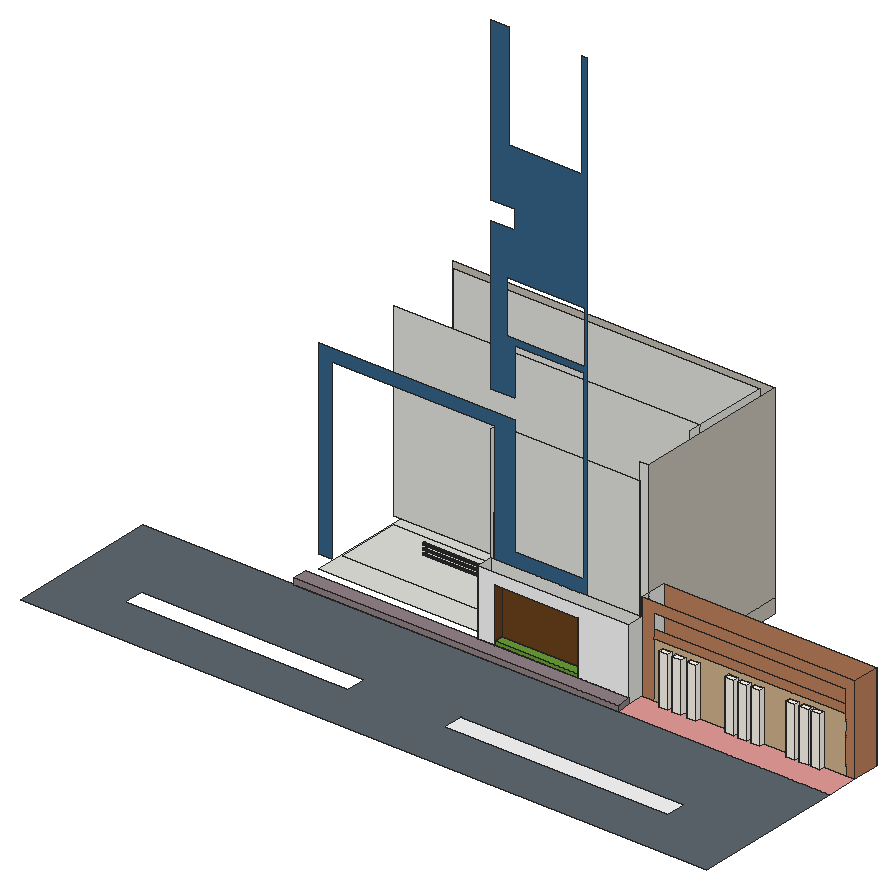
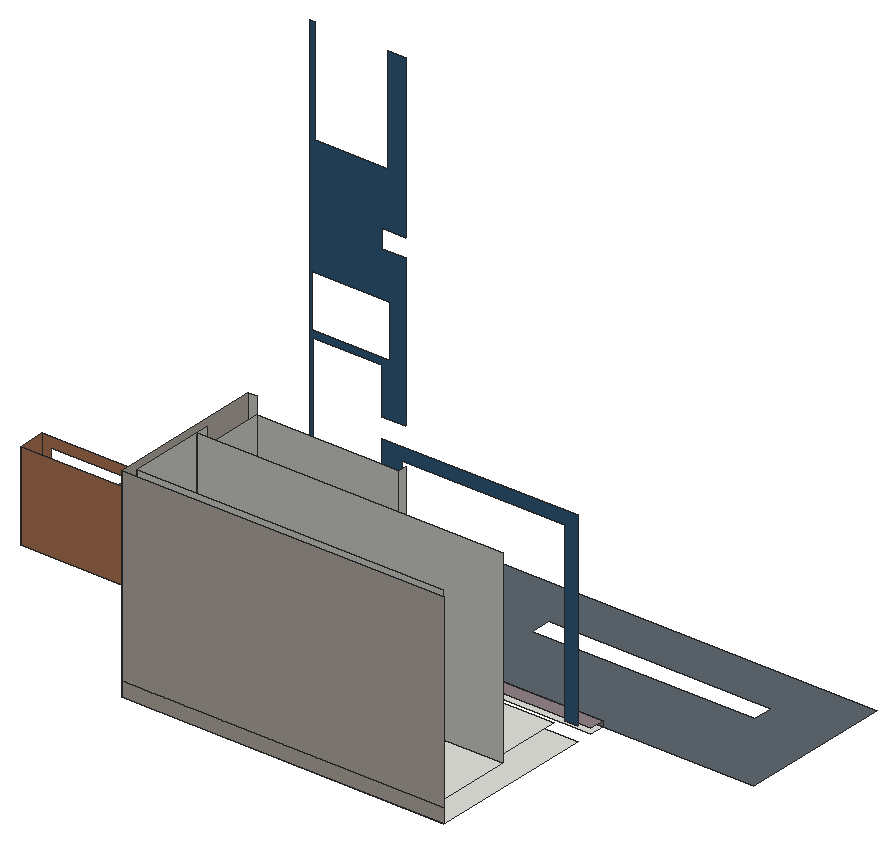
# SketchUp Ruby script. Lengths in inches.
U = 1.inch
M = Sketchup.active_model
def pt(a) = Geom::Point3d.new(a.map { |v| v * U })
def face(e, loops, mat)
  f = e.add_face(loops[0].map { |a| pt(a) })
  loops[1..].each { |l| e.add_face(l.map { |a| pt(a) }).erase! }
  f.material = f.back_material = mat if mat
  f
end
# faces: each face lists its corners as indices into pts; further lists are holes
def faces(e, pts, list, mat = nil) = list.each { |f| face(e, (f[0].is_a?(Array) ? f : [f]).map { |l| l.map { |i| pts[i] } }, mat) }
# xy, xz, yz: faces in a plane at the given z, y or x. An outline is a flat list of corners, or four numbers for a rectangle; further outlines are holes
def ring(l) = l.size == 4 ? [[l[0], l[1]], [l[2], l[1]], [l[2], l[3]], [l[0], l[3]]] : l.each_slice(2).to_a
def flat(e, list, mat, &to3) = list.each { |f| face(e, (f[0].is_a?(Array) ? f : [f]).map { |l| ring(l).map { |u, v| to3.(u, v) } }, mat) }
def xy(e, z, list, mat = nil) = flat(e, list, mat) { |x, y| [x, y, z] }
def xz(e, y, list, mat = nil) = flat(e, list, mat) { |x, z| [x, y, z] }
def yz(e, x, list, mat = nil) = flat(e, list, mat) { |y, z| [x, y, z] }
def lines(e, pts, list) = list.each { |a, b| e.add_line(pt(pts[a]), pt(pts[b])) }
# prism: a flat outline (further loops are holes) pulled along v
def prism(e, loops, v, mat = nil)
  f = face(e, loops, mat); d = Geom::Vector3d.new(v.map { |x| x * U })
  f.pushpull(f.normal.samedirection?(d) ? d.length : -d.length)
end
def box(e, o, s, mat = nil) = prism(e, [[o, [o[0] + s[0], o[1], o[2]], [o[0] + s[0], o[1] + s[1], o[2]], [o[0], o[1] + s[1], o[2]]]], [0, 0, s[2]], mat)
def at(x, y, z, deg = 0) = Geom::Transformation.translation(pt([x, y, z])) * Geom::Transformation.rotation(ORIGIN, Z_AXIS, deg.degrees)
def axes(o, x, y, z) = Geom::Transformation.new([*x, 0, *y, 0, *z, 0, *pt(o).to_a, 1])
def part(name) = M.definitions.add(name)
# library, detail: a bought-in or finely detailed component or shape, given as its bounding box
def library(name, o, s) = part(name).tap { |d| box(d.entities, o, s) }
def detail(e, o, s) = box(e.add_group.entities, o, s)
def put(e, d, t, mat = nil) = e.add_instance(d, t).tap { |i| i.material = mat if mat }
def group(e, t, mat = nil) = e.add_group.tap { |g| g.transformation = t; g.material = mat if mat }.entities
root = M.entities
M.materials.add("[0035_Tan]").color = [210, 180, 140]
M.materials.add("[0052_FloralWhite]").color = [255, 250, 240]
M.materials.add("[0100_SteelBlue]").color = [53, 99, 137]
M.materials.add("[Asphalt New]").color = [145, 130, 134]
M.materials.add("[Brick Basket]").color = [230, 156, 152]
M.materials.add("[Field Rectangle Tile]").color = [196, 189, 179]
M.materials.add("[Formica Laminate Dark]").color = [70, 74, 84]
M.materials.add("[Formica Speckled Grey]").color = [94, 105, 111]
M.materials.add("[Grass Dark Green]").color = [106, 157, 55]
M.materials.add("[Polished Concrete New]").color = [200, 200, 203]
M.materials.add("[Quartz Light Grey]").color = [251, 251, 252]
M.materials.add("[Wood Floor Parquet]").color = [107, 65, 28]
M.materials.add("[Wood Veneer 02]").color = [190, 128, 91]
xy(root,0,[[96.16,97.66,96.16,107.04,301.48,107.04,302.4,97.66],[205.34,107.04,205.34,117.35,301.48,117.35,301.48,107.04,269.29,107.04,269.29,112.73,216.35,112.73,216.35,107.04],[216.35,107.04,269.29,112.73],[315.22,114.1,320.97,117.35],[323.53,114.1,329.29,117.35],
  [332.72,114.1,338.47,117.35],[356.72,114.1,362.47,117.35],[365.41,114.1,371.16,117.35],[373.47,114.1,379.22,117.35],[396.03,114.1,401.79,117.35],
  [404.41,114.1,410.16,117.35],[411.78,114.1,417.54,117.35],[96.16,117.35,301.48,223.51],[301.48,117.35,437.01,134.6]])
xy(root,0,[[302.4,97.66,301.48,107.04,301.48,117.35,315.22,117.35,315.22,114.1,320.97,114.1,320.97,117.35,323.53,117.35,323.53,114.1,329.29,114.1,329.29,117.35,332.72,117.35,332.72,114.1,338.47,114.1,338.47,117.35,356.72,117.35,356.72,114.1,362.47,114.1,362.47,117.35,365.41,117.35,365.41,114.1,371.16,114.1,371.16,117.35,373.47,117.35,373.47,114.1,379.22,114.1,379.22,117.35,396.03,117.35,396.03,114.1,401.79,114.1,401.79,117.35,404.41,117.35,404.41,114.1,410.16,114.1,410.16,117.35,411.78,117.35,411.78,114.1,417.54,114.1,417.54,117.35,437.01,117.35,437.01,97.66]],"[Brick Basket]")
xy(root,0,[[[0,0,437.01,97.66],[41.43,31,183.87,44.5],[244.62,31,387.06,44.5]]],"[Formica Speckled Grey]")
xy(root,0,[[244.62,31,387.06,44.5]],"[Quartz Light Grey]")
xy(root,0.6875,[[216.35,107.04,269.29,112.73]],"[Wood Floor Parquet]")
xy(root,3.4375,[[96.16,97.66,302.4,97.66,301.48,107.04,96.16,107.04]],"[Asphalt New]")
xy(root,5.8125,[[216.35,107.04,269.29,112.73]],"[Grass Dark Green]")
xy(root,9,[[107.21,122.78,296.05,162.72],[101.58,170.43,296.05,218.08]])
xy(root,10.25,[[204.4,118.87,205.34,121.64]])
xy(root,31.59,[[315.22,114.1,320.97,117.35],[323.53,114.1,329.29,117.35],[332.72,114.1,338.47,117.35],[356.72,114.1,362.47,117.35],[365.41,114.1,371.16,117.35],
  [373.47,114.1,379.22,117.35],[396.03,114.1,401.79,117.35],[404.41,114.1,410.16,117.35],[411.78,114.1,417.54,117.35]],"[0052_FloralWhite]")
xz(root,97.66,[[96.16,0,302.4,3.4375]],"[Asphalt New]")
xz(root,107.04,[[205.34,0,216.35,3.4375],[216.35,0,269.29,0.6875],[269.29,0,301.48,3.4375],[216.35,0.6875,269.29,3.4375]])
xz(root,107.04,[[216.35,3.4375,269.29,5.8125]],"[Grass Dark Green]")
xz(root,107.04,[[205.34,3.4375,216.35,3.4375,216.35,37.8125,269.29,37.8125,269.29,3.4375,301.48,3.4375,301.48,44.875,205.34,44.875]],"[Quartz Light Grey]")
xz(root,112.73,[[216.35,0,269.29,0.6875]])
xz(root,112.73,[[216.35,0.6875,269.29,5.8125],[216.35,5.8125,269.29,37.8125]],"[Wood Floor Parquet]")
xz(root,114.1,[[315.22,0,320.97,31.59],[323.53,0,329.29,31.59],[332.72,0,338.47,31.59],[356.72,0,362.47,31.59],[365.41,0,371.16,31.59],
  [373.47,0,379.22,31.59],[396.03,0,401.79,31.59],[404.41,0,410.16,31.59],[411.78,0,417.54,31.59]],"[0052_FloralWhite]")
xz(root,117.35,[[205.34,0,301.48,44.875],[315.22,0,320.97,31.59],[323.53,0,329.29,31.59],[332.72,0,338.47,31.59],[356.72,0,362.47,31.59],
  [365.41,0,371.16,31.59],[373.47,0,379.22,31.59],[396.03,0,401.79,31.59],[404.41,0,410.16,31.59],[411.78,0,417.54,31.59]])
xz(root,117.35,[[309.46,0,315.22,0,315.22,31.59,320.97,31.59,320.97,0,323.53,0,323.53,31.59,329.29,31.59,329.29,0,332.72,0,332.72,31.59,338.47,31.59,338.47,0,356.72,0,356.72,31.59,362.47,31.59,362.47,0,365.41,0,365.41,31.59,371.16,31.59,371.16,0,373.47,0,373.47,31.59,379.22,31.59,379.22,0,396.03,0,396.03,31.59,401.79,31.59,401.79,0,404.41,0,404.41,31.59,410.16,31.59,410.16,0,411.78,0,411.78,31.59,417.54,31.59,417.54,0,431.59,0,431.59,35.47,309.46,35.47]],"[0035_Tan]")
xz(root,117.35,[[[96.16,9,104.33,9,104.33,120.875,207.77,120.875,207.77,44.875,266.37,44.875,266.37,351.35,263.15,351.35,263.15,284.16,216.72,284.16,216.72,351.35,205.34,351.35,205.34,249,220.625,249,220.625,237.17,205.34,237.17,205.34,141.375,220.625,141.375,220.625,171.19,264.66,171.19,264.66,53.88,220.625,53.88,220.625,129,96.16,129],[215.78,175.07,265.4,208.67]]],"[0100_SteelBlue]")
xz(root,117.35,[[301.48,0,309.46,0,309.46,49.875,431.59,49.875,431.59,0,437.01,0,437.01,56.125,301.48,56.125],[309.46,35.47,431.59,40.81]],"[Wood Veneer 02]")
xz(root,122.78,[[205.34,9,296.05,118.16],[296.05,9,301.48,129]])
xz(root,134.6,[[301.48,0,437.01,56.125]],"[Wood Veneer 02]")
xz(root,170.43,[[101.58,9,296.05,129]])
xz(root,218.08,[[101.58,9,296.05,129]])
xz(root,223.51,[[96.16,0,301.48,9],[96.16,9,301.48,129]],"[Field Rectangle Tile]")
yz(root,204.4,[[120.29,10.73,120.45,10.75,120.6,10.8125,120.73,10.91,120.83,11.04,120.89,11.19,120.91,11.35,120.89,11.51,120.83,11.66,120.73,11.79,120.6,11.89,120.45,11.96,120.29,11.98,120.13,11.96,119.98,11.89,119.85,11.79,119.75,11.66,119.6875,11.51,119.66,11.35,119.6875,11.19,119.75,11.04,119.85,10.91,119.98,10.8125,120.13,10.75],[120.29,13.16,120.45,13.1875,120.6,13.25,120.73,13.35,120.83,13.48,120.89,13.63,120.91,13.79,120.89,13.95,120.83,14.1,120.73,14.23,120.6,14.33,120.45,14.39,120.29,14.41,120.13,14.39,119.98,14.33,119.85,14.23,119.75,14.1,119.6875,13.95,119.66,13.79,119.6875,13.63,119.75,13.48,119.85,13.35,119.98,13.25,120.13,13.1875],[120.29,15.54,120.45,15.5625,120.6,15.625,120.73,15.72,120.83,15.85,120.89,16,120.91,16.16,120.89,16.33,120.83,16.48,120.73,16.61,120.6,16.71,120.45,16.77,120.29,16.79,120.13,16.77,119.98,16.71,119.85,16.61,119.75,16.48,119.6875,16.33,119.66,16.16,119.6875,16,119.75,15.85,119.85,15.72,119.98,15.625,120.13,15.5625],[120.29,17.91,120.45,17.9375,120.6,18,120.73,18.1,120.83,18.23,120.89,18.38,120.91,18.54,120.89,18.7,120.83,18.85,120.73,18.98,120.6,19.08,120.45,19.14,120.29,19.16,120.13,19.14,119.98,19.08,119.85,18.98,119.75,18.85,119.6875,18.7,119.66,18.54,119.6875,18.38,119.75,18.23,119.85,18.1,119.98,18,120.13,17.9375],[120.29,20.29,120.45,20.3125,120.6,20.375,120.73,20.47,120.83,20.6,120.89,20.75,120.91,20.91,120.89,21.08,120.83,21.23,120.73,21.36,120.6,21.46,120.45,21.52,120.29,21.54,120.13,21.52,119.98,21.46,119.85,21.36,119.75,21.23,119.6875,21.08,119.66,20.91,119.6875,20.75,119.75,20.6,119.85,20.47,119.98,20.375,120.13,20.3125],
  [120.29,22.48,120.45,22.5,120.6,22.5625,120.73,22.66,120.83,22.79,120.89,22.94,120.91,23.1,120.89,23.26,120.83,23.41,120.73,23.54,120.6,23.64,120.45,23.71,120.29,23.73,120.13,23.71,119.98,23.64,119.85,23.54,119.75,23.41,119.6875,23.26,119.66,23.1,119.6875,22.94,119.75,22.79,119.85,22.66,119.98,22.5625,120.13,22.5],[120.29,24.23,120.45,24.25,120.6,24.3125,120.73,24.41,120.83,24.54,120.89,24.69,120.91,24.85,120.89,25.01,120.83,25.16,120.73,25.29,120.6,25.39,120.45,25.46,120.29,25.48,120.13,25.46,119.98,25.39,119.85,25.29,119.75,25.16,119.6875,25.01,119.66,24.85,119.6875,24.69,119.75,24.54,119.85,24.41,119.98,24.3125,120.13,24.25],[120.29,26.41,120.45,26.4375,120.6,26.5,120.73,26.6,120.83,26.73,120.89,26.88,120.91,27.04,120.89,27.2,120.83,27.35,120.73,27.48,120.6,27.58,120.45,27.64,120.29,27.66,120.13,27.64,119.98,27.58,119.85,27.48,119.75,27.35,119.6875,27.2,119.66,27.04,119.6875,26.88,119.75,26.73,119.85,26.6,119.98,26.5,120.13,26.4375],[120.29,29.35,120.45,29.375,120.6,29.4375,120.73,29.54,120.83,29.66,120.89,29.82,120.91,29.98,120.89,30.14,120.83,30.29,120.73,30.42,120.6,30.52,120.45,30.58,120.29,30.6,120.13,30.58,119.98,30.52,119.85,30.42,119.75,30.29,119.6875,30.14,119.66,29.98,119.6875,29.82,119.75,29.66,119.85,29.54,119.98,29.4375,120.13,29.375],[120.29,32.16,120.45,32.1875,120.6,32.25,120.73,32.35,120.83,32.48,120.89,32.63,120.91,32.79,120.89,32.95,120.83,33.1,120.73,33.23,120.6,33.33,120.45,33.39,120.29,33.41,120.13,33.39,119.98,33.33,119.85,33.23,119.75,33.1,119.6875,32.95,119.66,32.79,119.6875,32.63,119.75,32.48,119.85,32.35,119.98,32.25,120.13,32.1875],
  [120.29,35.29,120.45,35.3125,120.6,35.375,120.73,35.47,120.83,35.6,120.89,35.75,120.91,35.91,120.89,36.08,120.83,36.23,120.73,36.36,120.6,36.46,120.45,36.52,120.29,36.54,120.13,36.52,119.98,36.46,119.85,36.36,119.75,36.23,119.6875,36.08,119.66,35.91,119.6875,35.75,119.75,35.6,119.85,35.47,119.98,35.375,120.13,35.3125]])
yz(root,204.4,[[[118.87,10.25,121.64,67.58],[120.29,15.54,120.45,15.5625,120.6,15.625,120.73,15.72,120.83,15.85,120.89,16,120.91,16.16,120.89,16.33,120.83,16.48,120.73,16.61,120.6,16.71,120.45,16.77,120.29,16.79,120.13,16.77,119.98,16.71,119.85,16.61,119.75,16.48,119.6875,16.33,119.66,16.16,119.6875,16,119.75,15.85,119.85,15.72,119.98,15.625,120.13,15.5625],[120.29,63.23,120.45,63.25,120.6,63.3125,120.73,63.41,120.83,63.54,120.89,63.69,120.91,63.85,120.89,64.01,120.83,64.16,120.73,64.29,120.6,64.39,120.45,64.46,120.29,64.48,120.13,64.46,119.98,64.39,119.85,64.29,119.75,64.16,119.6875,64.01,119.66,63.85,119.6875,63.69,119.75,63.54,119.85,63.41,119.98,63.3125,120.13,63.25],[120.29,65.54,120.45,65.5625,120.6,65.625,120.73,65.72,120.83,65.85,120.89,66,120.91,66.16,120.89,66.33,120.83,66.48,120.73,66.61,120.6,66.71,120.45,66.77,120.29,66.79,120.13,66.77,119.98,66.71,119.85,66.61,119.75,66.48,119.6875,66.33,119.66,66.16,119.6875,66,119.75,65.85,119.85,65.72,119.98,65.625,120.13,65.5625],[120.29,10.73,120.45,10.75,120.6,10.8125,120.73,10.91,120.83,11.04,120.89,11.19,120.91,11.35,120.89,11.51,120.83,11.66,120.73,11.79,120.6,11.89,120.45,11.96,120.29,11.98,120.13,11.96,119.98,11.89,119.85,11.79,119.75,11.66,119.6875,11.51,119.66,11.35,119.6875,11.19,119.75,11.04,119.85,10.91,119.98,10.8125,120.13,10.75],[120.29,13.16,120.45,13.1875,120.6,13.25,120.73,13.35,120.83,13.48,120.89,13.63,120.91,13.79,120.89,13.95,120.83,14.1,120.73,14.23,120.6,14.33,120.45,14.39,120.29,14.41,120.13,14.39,119.98,14.33,119.85,14.23,119.75,14.1,119.6875,13.95,119.66,13.79,119.6875,13.63,119.75,13.48,119.85,13.35,119.98,13.25,120.13,13.1875],[120.29,17.91,120.45,17.9375,120.6,18,120.73,18.1,120.83,18.23,120.89,18.38,120.91,18.54,120.89,18.7,120.83,18.85,120.73,18.98,120.6,19.08,120.45,19.14,120.29,19.16,120.13,19.14,119.98,19.08,119.85,18.98,119.75,18.85,119.6875,18.7,119.66,18.54,119.6875,18.38,119.75,18.23,119.85,18.1,119.98,18,120.13,17.9375],[120.29,20.29,120.45,20.3125,120.6,20.375,120.73,20.47,120.83,20.6,120.89,20.75,120.91,20.91,120.89,21.08,120.83,21.23,120.73,21.36,120.6,21.46,120.45,21.52,120.29,21.54,120.13,21.52,119.98,21.46,119.85,21.36,119.75,21.23,119.6875,21.08,119.66,20.91,119.6875,20.75,119.75,20.6,119.85,20.47,119.98,20.375,120.13,20.3125],[120.29,22.48,120.45,22.5,120.6,22.5625,120.73,22.66,120.83,22.79,120.89,22.94,120.91,23.1,120.89,23.26,120.83,23.41,120.73,23.54,120.6,23.64,120.45,23.71,120.29,23.73,120.13,23.71,119.98,23.64,119.85,23.54,119.75,23.41,119.6875,23.26,119.66,23.1,119.6875,22.94,119.75,22.79,119.85,22.66,119.98,22.5625,120.13,22.5],[120.29,24.23,120.45,24.25,120.6,24.3125,120.73,24.41,120.83,24.54,120.89,24.69,120.91,24.85,120.89,25.01,120.83,25.16,120.73,25.29,120.6,25.39,120.45,25.46,120.29,25.48,120.13,25.46,119.98,25.39,119.85,25.29,119.75,25.16,119.6875,25.01,119.66,24.85,119.6875,24.69,119.75,24.54,119.85,24.41,119.98,24.3125,120.13,24.25],[120.29,26.41,120.45,26.4375,120.6,26.5,120.73,26.6,120.83,26.73,120.89,26.88,120.91,27.04,120.89,27.2,120.83,27.35,120.73,27.48,120.6,27.58,120.45,27.64,120.29,27.66,120.13,27.64,119.98,27.58,119.85,27.48,119.75,27.35,119.6875,27.2,119.66,27.04,119.6875,26.88,119.75,26.73,119.85,26.6,119.98,26.5,120.13,26.4375],[120.29,29.35,120.45,29.375,120.6,29.4375,120.73,29.54,120.83,29.66,120.89,29.82,120.91,29.98,120.89,30.14,120.83,30.29,120.73,30.42,120.6,30.52,120.45,30.58,120.29,30.6,120.13,30.58,119.98,30.52,119.85,30.42,119.75,30.29,119.6875,30.14,119.66,29.98,119.6875,29.82,119.75,29.66,119.85,29.54,119.98,29.4375,120.13,29.375],[120.29,32.16,120.45,32.1875,120.6,32.25,120.73,32.35,120.83,32.48,120.89,32.63,120.91,32.79,120.89,32.95,120.83,33.1,120.73,33.23,120.6,33.33,120.45,33.39,120.29,33.41,120.13,33.39,119.98,33.33,119.85,33.23,119.75,33.1,119.6875,32.95,119.66,32.79,119.6875,32.63,119.75,32.48,119.85,32.35,119.98,32.25,120.13,32.1875],[120.29,35.29,120.45,35.3125,120.6,35.375,120.73,35.47,120.83,35.6,120.89,35.75,120.91,35.91,120.89,36.08,120.83,36.23,120.73,36.36,120.6,36.46,120.45,36.52,120.29,36.54,120.13,36.52,119.98,36.46,119.85,36.36,119.75,36.23,119.6875,36.08,119.66,35.91,119.6875,35.75,119.75,35.6,119.85,35.47,119.98,35.375,120.13,35.3125],[120.29,38.04,120.45,38.0625,120.6,38.125,120.73,38.22,120.83,38.35,120.89,38.5,120.91,38.66,120.89,38.83,120.83,38.98,120.73,39.11,120.6,39.21,120.45,39.27,120.29,39.29,120.13,39.27,119.98,39.21,119.85,39.11,119.75,38.98,119.6875,38.83,119.66,38.66,119.6875,38.5,119.75,38.35,119.85,38.22,119.98,38.125,120.13,38.0625],[120.29,41.04,120.45,41.0625,120.6,41.125,120.73,41.22,120.83,41.35,120.89,41.5,120.91,41.66,120.89,41.83,120.83,41.98,120.73,42.11,120.6,42.21,120.45,42.27,120.29,42.29,120.13,42.27,119.98,42.21,119.85,42.11,119.75,41.98,119.6875,41.83,119.66,41.66,119.6875,41.5,119.75,41.35,119.85,41.22,119.98,41.125,120.13,41.0625],[120.29,43.91,120.45,43.9375,120.6,44,120.73,44.1,120.83,44.23,120.89,44.38,120.91,44.54,120.89,44.7,120.83,44.85,120.73,44.98,120.6,45.08,120.45,45.14,120.29,45.16,120.13,45.14,119.98,45.08,119.85,44.98,119.75,44.85,119.6875,44.7,119.66,44.54,119.6875,44.38,119.75,44.23,119.85,44.1,119.98,44,120.13,43.9375],[120.29,47.41,120.45,47.4375,120.6,47.5,120.73,47.6,120.83,47.73,120.89,47.88,120.91,48.04,120.89,48.2,120.83,48.35,120.73,48.48,120.6,48.58,120.45,48.64,120.29,48.66,120.13,48.64,119.98,48.58,119.85,48.48,119.75,48.35,119.6875,48.2,119.66,48.04,119.6875,47.88,119.75,47.73,119.85,47.6,119.98,47.5,120.13,47.4375],[120.29,50.29,120.45,50.3125,120.6,50.375,120.73,50.47,120.83,50.6,120.89,50.75,120.91,50.91,120.89,51.08,120.83,51.23,120.73,51.36,120.6,51.46,120.45,51.52,120.29,51.54,120.13,51.52,119.98,51.46,119.85,51.36,119.75,51.23,119.6875,51.08,119.66,50.91,119.6875,50.75,119.75,50.6,119.85,50.47,119.98,50.375,120.13,50.3125],[120.29,53.35,120.45,53.375,120.6,53.4375,120.73,53.54,120.83,53.66,120.89,53.82,120.91,53.98,120.89,54.14,120.83,54.29,120.73,54.42,120.6,54.52,120.45,54.58,120.29,54.6,120.13,54.58,119.98,54.52,119.85,54.42,119.75,54.29,119.6875,54.14,119.66,53.98,119.6875,53.82,119.75,53.66,119.85,53.54,119.98,53.4375,120.13,53.375],[120.29,55.6,120.45,55.625,120.6,55.6875,120.73,55.79,120.83,55.91,120.89,56.07,120.91,56.23,120.89,56.39,120.83,56.54,120.73,56.67,120.6,56.77,120.45,56.83,120.29,56.85,120.13,56.83,119.98,56.77,119.85,56.67,119.75,56.54,119.6875,56.39,119.66,56.23,119.6875,56.07,119.75,55.91,119.85,55.79,119.98,55.6875,120.13,55.625],[120.29,58.16,120.45,58.1875,120.6,58.25,120.73,58.35,120.83,58.48,120.89,58.63,120.91,58.79,120.89,58.95,120.83,59.1,120.73,59.23,120.6,59.33,120.45,59.39,120.29,59.41,120.13,59.39,119.98,59.33,119.85,59.23,119.75,59.1,119.6875,58.95,119.66,58.79,119.6875,58.63,119.75,58.48,119.85,58.35,119.98,58.25,120.13,58.1875],[120.29,60.85,120.45,60.875,120.6,60.9375,120.73,61.04,120.83,61.16,120.89,61.32,120.91,61.48,120.89,61.64,120.83,61.79,120.73,61.92,120.6,62.02,120.45,62.08,120.29,62.1,120.13,62.08,119.98,62.02,119.85,61.92,119.75,61.79,119.6875,61.64,119.66,61.48,119.6875,61.32,119.75,61.16,119.85,61.04,119.98,60.9375,120.13,60.875]]],"[Formica Laminate Dark]")
yz(root,205.34,[[107.04,0,117.35,9],[107.04,9,117.35,44.875],[117.35,9,117.35,118.16,122.78,118.16,122.78,9,121.64,9,121.64,69.75,118.87,69.75,118.87,9],[118.87,9,121.64,10.25],[118.87,10.25,121.64,69.75]])
yz(root,216.35,[[107.04,0,112.73,0.6875]])
yz(root,216.35,[[107.04,0.6875,112.73,5.8125],[107.04,5.8125,112.73,37.8125]],"[Wood Floor Parquet]")
yz(root,269.29,[[107.04,0,112.73,0.6875]])
yz(root,269.29,[[107.04,0.6875,112.73,5.8125],[107.04,5.8125,112.73,37.8125]],"[Wood Floor Parquet]")
yz(root,296.05,[[122.78,9,162.72,118.16],[162.72,9,170.43,129],[170.43,9,218.08,129]])
yz(root,301.48,[[107.04,0,117.35,44.875],[117.35,0,117.35,56.125,122.78,56.125,122.78,9,134.6,9,134.6,0],[122.78,9,134.6,56.125]])
yz(root,301.48,[[134.6,0,223.51,9],[134.6,9,223.51,9,223.51,129,122.78,129,122.78,56.125,134.6,56.125]],"[Field Rectangle Tile]")
yz(root,315.22,[[114.1,0,117.35,31.59]],"[0052_FloralWhite]")
yz(root,320.97,[[114.1,0,117.35,31.59]],"[0052_FloralWhite]")
yz(root,323.53,[[114.1,0,117.35,31.59]],"[0052_FloralWhite]")
yz(root,329.29,[[114.1,0,117.35,31.59]],"[0052_FloralWhite]")
yz(root,332.72,[[114.1,0,117.35,31.59]],"[0052_FloralWhite]")
yz(root,338.47,[[114.1,0,117.35,31.59]],"[0052_FloralWhite]")
yz(root,356.72,[[114.1,0,117.35,31.59]],"[0052_FloralWhite]")
yz(root,362.47,[[114.1,0,117.35,31.59]],"[0052_FloralWhite]")
yz(root,365.41,[[114.1,0,117.35,31.59]],"[0052_FloralWhite]")
yz(root,371.16,[[114.1,0,117.35,31.59]],"[0052_FloralWhite]")
yz(root,373.47,[[114.1,0,117.35,31.59]],"[0052_FloralWhite]")
yz(root,379.22,[[114.1,0,117.35,31.59]],"[0052_FloralWhite]")
yz(root,396.03,[[114.1,0,117.35,31.59]],"[0052_FloralWhite]")
yz(root,401.79,[[114.1,0,117.35,31.59]],"[0052_FloralWhite]")
yz(root,404.41,[[114.1,0,117.35,31.59]],"[0052_FloralWhite]")
yz(root,410.16,[[114.1,0,117.35,31.59]],"[0052_FloralWhite]")
yz(root,411.78,[[114.1,0,117.35,31.59]],"[0052_FloralWhite]")
yz(root,417.54,[[114.1,0,117.35,31.59]],"[0052_FloralWhite]")
yz(root,437.01,[[117.35,0,134.6,56.125]],"[Wood Veneer 02]")
p = [[302.4,97.66,0],[301.48,107.04,0],[301.48,107.04,3.4375],[302.4,97.66,3.4375],[204.4,119.98,29.4375],[204.4,119.85,29.54],
  [160.24,119.85,29.54],[160.24,119.98,29.4375],[204.4,120.13,29.375],[160.24,120.13,29.375],[204.4,120.29,29.35],[160.24,120.29,29.35],
  [204.4,120.6,29.4375],[204.4,120.45,29.375],[160.24,120.45,29.375],[160.24,120.6,29.4375],[204.4,120.73,29.54],[160.24,120.73,29.54],
  [204.4,119.75,29.66],[160.24,119.75,29.66],[204.4,120.83,29.66],[160.24,120.83,29.66],[204.4,119.6875,29.82],[160.24,119.6875,29.82],
  [204.4,120.89,29.82],[160.24,120.89,29.82],[204.4,119.66,29.98],[160.24,119.66,29.98],[204.4,120.91,29.98],[160.24,120.91,29.98],
  [204.4,119.6875,30.14],[160.24,119.6875,30.14],[204.4,120.89,30.14],[160.24,120.89,30.14],[204.4,119.75,30.29],[160.24,119.75,30.29],
  [204.4,120.83,30.29],[160.24,120.83,30.29],[204.4,119.85,30.42],[160.24,119.85,30.42],[204.4,120.73,30.42],[160.24,120.73,30.42],
  [204.4,119.98,30.52],[160.24,119.98,30.52],[204.4,120.6,30.52],[160.24,120.6,30.52],[204.4,120.13,30.58],[160.24,120.13,30.58],
  [204.4,120.45,30.58],[160.24,120.45,30.58],[204.4,120.29,30.6],[160.24,120.29,30.6],[204.4,119.98,32.25],[204.4,119.85,32.35],
  [160.24,119.85,32.35],[160.24,119.98,32.25],[204.4,120.13,32.1875],[160.24,120.13,32.1875],[204.4,120.29,32.16],[160.24,120.29,32.16],
  [204.4,120.45,32.1875],[160.24,120.45,32.1875],[204.4,120.6,32.25],[160.24,120.6,32.25],[204.4,120.73,32.35],[160.24,120.73,32.35],
  [204.4,119.75,32.48],[160.24,119.75,32.48],[204.4,120.83,32.48],[160.24,120.83,32.48],[204.4,119.6875,32.63],[160.24,119.6875,32.63],
  [204.4,120.89,32.63],[160.24,120.89,32.63],[204.4,119.66,32.79],[160.24,119.66,32.79],[204.4,120.91,32.79],[160.24,120.91,32.79],
  [204.4,119.6875,32.95],[160.24,119.6875,32.95],[204.4,120.89,32.95],[160.24,120.89,32.95],[204.4,119.75,33.1],[160.24,119.75,33.1],
  [204.4,120.83,33.1],[160.24,120.83,33.1],[204.4,119.85,33.23],[160.24,119.85,33.23],[204.4,120.73,33.23],[160.24,120.73,33.23],
  [204.4,119.98,33.33],[160.24,119.98,33.33],[204.4,120.6,33.33],[160.24,120.6,33.33],[204.4,120.13,33.39],[160.24,120.13,33.39],
  [204.4,120.45,33.39],[160.24,120.45,33.39],[204.4,120.29,33.41],[160.24,120.29,33.41],[204.4,120.13,35.3125],[204.4,119.98,35.375],
  [160.24,119.98,35.375],[160.24,120.13,35.3125],[204.4,120.29,35.29],[160.24,120.29,35.29],[204.4,120.45,35.3125],[160.24,120.45,35.3125],
  [204.4,120.6,35.375],[160.24,120.6,35.375],[204.4,119.85,35.47],[160.24,119.85,35.47],[204.4,120.73,35.47],[160.24,120.73,35.47],
  [204.4,119.75,35.6],[160.24,119.75,35.6],[204.4,120.83,35.6],[160.24,120.83,35.6],[204.4,119.6875,35.75],[160.24,119.6875,35.75],
  [204.4,120.89,35.75],[160.24,120.89,35.75],[204.4,119.66,35.91],[160.24,119.66,35.91],[204.4,120.91,35.91],[160.24,120.91,35.91],
  [204.4,119.6875,36.08],[160.24,119.6875,36.08],[204.4,120.89,36.08],[160.24,120.89,36.08],[204.4,119.75,36.23],[160.24,119.75,36.23],
  [204.4,120.83,36.23],[160.24,120.83,36.23],[204.4,119.85,36.36],[160.24,119.85,36.36],[204.4,120.73,36.36],[160.24,120.73,36.36],
  [204.4,119.98,36.46],[160.24,119.98,36.46],[204.4,120.6,36.46],[160.24,120.6,36.46],[204.4,120.13,36.52],[160.24,120.13,36.52],
  [204.4,120.29,36.54],[160.24,120.29,36.54],[204.4,120.45,36.52],[160.24,120.45,36.52]]
faces(root,p,[[0,1,2,3]],"[Asphalt New]")
faces(root,p,[[4,5,6,7],[8,4,7,9],[10,8,9,11],[12,13,14,15],[16,12,15,17],[5,18,19,6],[20,16,17,21],[18,22,23,19],
  [24,20,21,25],[22,26,27,23],[28,24,25,29],[26,30,31,27],[32,28,29,33],[30,34,35,31],[36,32,33,37],[34,38,39,35],
  [40,36,37,41],[38,42,43,39],[44,40,41,45],[42,46,47,43],[48,44,45,49],[46,50,51,47],[50,48,49,51],[52,53,54,55],
  [56,52,55,57],[58,56,57,59],[60,58,59,61],[62,60,61,63],[64,62,63,65],[53,66,67,54],[68,64,65,69],[66,70,71,67],
  [72,68,69,73],[70,74,75,71],[76,72,73,77],[74,78,79,75],[80,76,77,81],[78,82,83,79],[84,80,81,85],[82,86,87,83],
  [88,84,85,89],[86,90,91,87],[92,88,89,93],[90,94,95,91],[96,92,93,97],[94,98,99,95],[98,96,97,99],[100,101,102,103],
  [104,100,103,105],[106,104,105,107],[108,106,107,109],[101,110,111,102],[112,108,109,113],[110,114,115,111],[116,112,113,117],[114,118,119,115],
  [120,116,117,121],[118,122,123,119],[124,120,121,125],[122,126,127,123],[128,124,125,129],[126,130,131,127],[132,128,129,133],[130,134,135,131],
  [136,132,133,137],[134,138,139,135],[140,136,137,141],[138,142,143,139],[142,144,145,143],[144,146,147,145],[146,140,141,147]],"[Polished Concrete New]")
